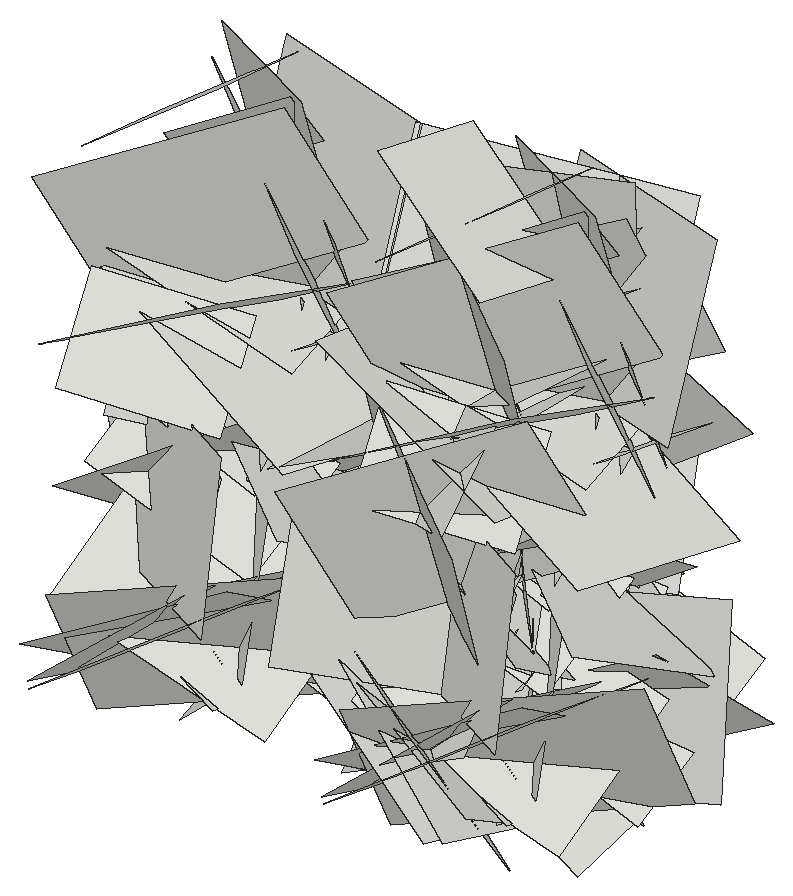
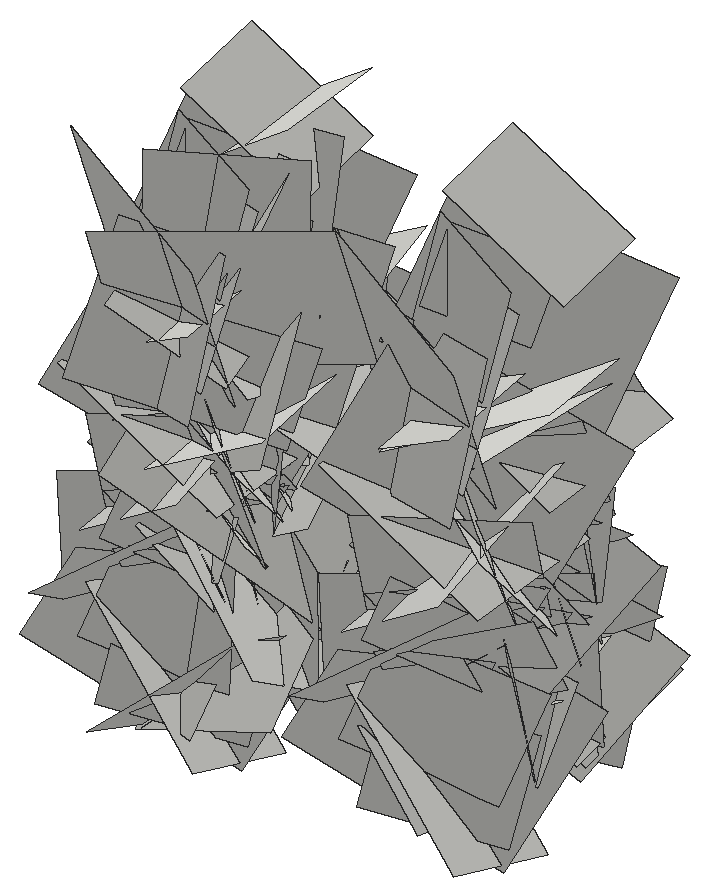
# SketchUp Ruby script. Lengths in inches.
U = 1.inch
M = Sketchup.active_model
def pt(a) = Geom::Point3d.new(a.map { |v| v * U })
def face(e, loops, mat)
  f = e.add_face(loops[0].map { |a| pt(a) })
  loops[1..].each { |l| e.add_face(l.map { |a| pt(a) }).erase! }
  f.material = f.back_material = mat if mat
  f
end
# faces: each face lists its corners as indices into pts; further lists are holes
def faces(e, pts, list, mat = nil) = list.each { |f| face(e, (f[0].is_a?(Array) ? f : [f]).map { |l| l.map { |i| pts[i] } }, mat) }
# xy, xz, yz: faces in a plane at the given z, y or x. An outline is a flat list of corners, or four numbers for a rectangle; further outlines are holes
def ring(l) = l.size == 4 ? [[l[0], l[1]], [l[2], l[1]], [l[2], l[3]], [l[0], l[3]]] : l.each_slice(2).to_a
def flat(e, list, mat, &to3) = list.each { |f| face(e, (f[0].is_a?(Array) ? f : [f]).map { |l| ring(l).map { |u, v| to3.(u, v) } }, mat) }
def xy(e, z, list, mat = nil) = flat(e, list, mat) { |x, y| [x, y, z] }
def xz(e, y, list, mat = nil) = flat(e, list, mat) { |x, z| [x, y, z] }
def yz(e, x, list, mat = nil) = flat(e, list, mat) { |y, z| [x, y, z] }
def lines(e, pts, list) = list.each { |a, b| e.add_line(pt(pts[a]), pt(pts[b])) }
# prism: a flat outline (further loops are holes) pulled along v
def prism(e, loops, v, mat = nil)
  f = face(e, loops, mat); d = Geom::Vector3d.new(v.map { |x| x * U })
  f.pushpull(f.normal.samedirection?(d) ? d.length : -d.length)
end
def box(e, o, s, mat = nil) = prism(e, [[o, [o[0] + s[0], o[1], o[2]], [o[0] + s[0], o[1] + s[1], o[2]], [o[0], o[1] + s[1], o[2]]]], [0, 0, s[2]], mat)
def at(x, y, z, deg = 0) = Geom::Transformation.translation(pt([x, y, z])) * Geom::Transformation.rotation(ORIGIN, Z_AXIS, deg.degrees)
def axes(o, x, y, z) = Geom::Transformation.new([*x, 0, *y, 0, *z, 0, *pt(o).to_a, 1])
def part(name) = M.definitions.add(name)
# library, detail: a bought-in or finely detailed component or shape, given as its bounding box
def library(name, o, s) = part(name).tap { |d| box(d.entities, o, s) }
def detail(e, o, s) = box(e.add_group.entities, o, s)
def put(e, d, t, mat = nil) = e.add_instance(d, t).tap { |i| i.material = mat if mat }
def group(e, t, mat = nil) = e.add_group.tap { |g| g.transformation = t; g.material = mat if mat }.entities
root = M.entities
c1 = part("Component\#6")
p = [[0.01,0,0],[0,3.24,4.54],[4.32,3.24,4.54],[4.33,0,0]]
faces(c1.entities,p,[[0,1,2,3]])
put(root,c1,axes([424.49,131.21,27.63],[0.2234,-0.54463,1.08834],[0.02633,1.10624,0.54877],[-1.28976,-0.07175,0.19972]))
put(root,c1,axes([420.52,131.21,27.63],[-0.2234,-0.54463,1.08834],[-0.02633,1.10624,0.54877],[1.28976,-0.07175,0.19972]))
put(root,c1,axes([410.71,134.27,30.6],[0.0256,-0.22889,-1.14247],[0.00761,-1.14266,0.22909],[1.23506,0.01178,0.02227]))
put(root,c1,axes([420.52,134.27,30.6],[0.0256,-0.22889,-1.14247],[0.00761,-1.14266,0.22909],[1.23506,0.01178,0.02227]))
put(root,c1,axes([424.49,134.27,30.6],[-0.0256,-0.22889,-1.14247],[-0.00761,-1.14266,0.22909],[-1.23506,0.01178,0.02227]))
put(root,c1,axes([420.52,134.18,33.55],[-0.07538,-0.44425,-0.62436],[0.04133,-0.62833,0.44263],[0.8112,-0.00926,-0.08057]))
put(root,c1,axes([414.68,134.18,33.55],[0.07538,-0.44425,-0.62436],[-0.04133,-0.62833,0.44263],[-0.8112,-0.00926,-0.08057]))
put(root,c1,axes([424.49,134.18,33.55],[0.07538,-0.44425,-0.62436],[-0.04133,-0.62833,0.44263],[-0.8112,-0.00926,-0.08057]))
put(root,c1,axes([410.71,134.17,21.91],[-0.00769,-1.04417,0.30366],[-0.13881,0.30229,1.03635],[1.14428,0.02965,0.12776]))
put(root,c1,axes([420.52,134.17,21.91],[-0.00769,-1.04417,0.30366],[-0.13881,0.30229,1.03635],[1.14428,0.02965,0.12776]))
put(root,c1,axes([424.49,134.17,21.91],[0.00769,-1.04417,0.30366],[0.13881,0.30229,1.03635],[-1.14428,0.02965,0.12776]))
put(root,c1,axes([410.71,134.58,22.11],[0.07114,-1.22092,0.271],[-0.02912,0.26988,1.2227],[1.32535,0.07146,0.01232]))
put(root,c1,axes([424.49,134.58,22.11],[-0.07114,-1.22092,0.271],[0.02912,0.26988,1.2227],[-1.32535,0.07146,0.01232]))
put(root,c1,axes([420.52,134.58,22.11],[0.07114,-1.22092,0.271],[-0.02912,0.26988,1.2227],[1.32535,0.07146,0.01232]))
put(root,c1,axes([410.71,134.42,21.5625],[-0.1234,-1.02964,0.56694],[0.11588,0.55776,1.03542],[1.24053,-0.15452,-0.04032]))
put(root,c1,axes([420.52,134.42,21.5625],[-0.1234,-1.02964,0.56694],[0.11588,0.55776,1.03542],[1.24053,-0.15452,-0.04032]))
put(root,c1,axes([424.49,134.42,21.5625],[0.1234,-1.02964,0.56694],[-0.11588,0.55776,1.03542],[-1.24053,-0.15452,-0.04032]))
put(root,c1,axes([410.71,132.49,21.15],[0.19066,-0.73145,1.17679],[0.11238,1.19045,0.72374],[1.46442,0.00387,-0.20876]))
put(root,c1,axes([420.52,132.49,21.15],[0.19066,-0.73145,1.17679],[0.11238,1.19045,0.72374],[1.46442,0.00387,-0.20876]))
put(root,c1,axes([424.49,132.49,21.15],[-0.19066,-0.73145,1.17679],[-0.11238,1.19045,0.72374],[-1.46442,0.00387,-0.20876]))
put(root,c1,axes([420.52,134.6875,22.2],[-0.10426,-0.66856,0.17597],[0.06243,0.169,0.67497],[0.73015,-0.10992,-0.03258]))
put(root,c1,axes([414.68,134.6875,22.2],[0.10426,-0.66856,0.17597],[-0.06243,0.169,0.67497],[-0.73015,-0.10992,-0.03258]))
put(root,c1,axes([424.49,134.6875,22.2],[0.10426,-0.66856,0.17597],[-0.06243,0.169,0.67497],[-0.73015,-0.10992,-0.03258]))
put(root,c1,axes([414.68,131.06,25.92],[0.11704,0.23417,0.88186],[0.10525,0.87993,-0.24609],[-0.96142,0.12483,0.08041]))
put(root,c1,axes([420.52,131.06,25.92],[-0.11704,0.23417,0.88186],[-0.10525,0.87993,-0.24609],[0.96142,0.12483,0.08041]))
put(root,c1,axes([424.49,131.06,25.92],[0.11704,0.23417,0.88186],[0.10525,0.87993,-0.24609],[-0.96142,0.12483,0.08041]))
put(root,c1,axes([410.71,130.54,25.39],[0.14552,0.87979,0.74939],[0.0105,0.75374,-0.8867],[1.22498,-0.11098,-0.08143]))
put(root,c1,axes([420.52,130.54,25.39],[0.14552,0.87979,0.74939],[0.0105,0.75374,-0.8867],[1.22498,-0.11098,-0.08143]))
put(root,c1,axes([424.49,130.54,25.39],[-0.14552,0.87979,0.74939],[-0.0105,0.75374,-0.8867],[-1.22498,-0.11098,-0.08143]))
put(root,c1,axes([410.71,135.84,31.22],[-0.16391,-1.12855,0.28901],[0.13375,0.27361,1.13591],[1.2276,-0.1805,-0.08517]))
put(root,c1,axes([420.52,135.84,31.22],[-0.16391,-1.12855,0.28901],[0.13375,0.27361,1.13591],[1.2276,-0.1805,-0.08517]))
put(root,c1,axes([424.49,135.84,31.22],[0.16391,-1.12855,0.28901],[-0.13375,0.27361,1.13591],[-1.2276,-0.1805,-0.08517]))
put(root,c1,axes([410.71,135.18,37.85],[0.05885,-0.83818,0.13983],[-0.03078,0.13818,0.83979],[0.90022,0.05952,0.01957]))
put(root,c1,axes([420.52,135.18,37.85],[0.05885,-0.83818,0.13983],[-0.03078,0.13818,0.83979],[0.90022,0.05952,0.01957]))
put(root,c1,axes([424.49,135.18,37.85],[-0.05885,-0.83818,0.13983],[0.03078,0.13818,0.83979],[-0.90022,0.05952,0.01957]))
put(root,c1,axes([410.71,133.37,32.625],[-0.2234,-0.54463,1.08834],[-0.02633,1.10624,0.54877],[1.28976,-0.07175,0.19972]))
put(root,c1,axes([424.49,133.37,32.625],[0.2234,-0.54463,1.08834],[0.02633,1.10624,0.54877],[-1.28976,-0.07175,0.19972]))
put(root,c1,axes([420.52,133.37,32.625],[-0.2234,-0.54463,1.08834],[-0.02633,1.10624,0.54877],[1.28976,-0.07175,0.19972]))
put(root,c1,axes([410.71,131.97,28.78],[0.10091,0.74431,0.53228],[-0.01265,0.53611,-0.74754],[0.96987,-0.07045,-0.06513]))
put(root,c1,axes([420.52,131.97,28.78],[0.10091,0.74431,0.53228],[-0.01265,0.53611,-0.74754],[0.96987,-0.07045,-0.06513]))
put(root,c1,axes([424.49,131.97,28.78],[-0.10091,0.74431,0.53228],[0.01265,0.53611,-0.74754],[-0.96987,-0.07045,-0.06513]))
put(root,c1,axes([414.68,136.41,29.65],[0.07813,-0.63244,-0.26103],[0.10098,-0.25049,0.63382],[-0.71818,-0.10402,0.06072]))
put(root,c1,axes([420.52,136.41,29.65],[-0.07813,-0.63244,-0.26103],[-0.10098,-0.25049,0.63382],[0.71818,-0.10402,0.06072]))
put(root,c1,axes([424.49,136.41,29.65],[0.07813,-0.63244,-0.26103],[0.10098,-0.25049,0.63382],[-0.71818,-0.10402,0.06072]))
put(root,c1,axes([410.71,134.54,24.9375],[0.02484,0.40022,-0.64969],[0.07983,-0.64803,-0.39648],[0.8049,0.05192,0.05937]))
put(root,c1,axes([420.52,134.54,24.9375],[0.02484,0.40022,-0.64969],[0.07983,-0.64803,-0.39648],[0.8049,0.05192,0.05937]))
put(root,c1,axes([424.49,134.54,24.9375],[-0.02484,0.40022,-0.64969],[-0.07983,-0.64803,-0.39648],[-0.8049,0.05192,0.05937]))
put(root,c1,axes([410.71,136.25,25.03],[-0.1909,-1.05424,0.65515],[0.04228,0.65676,1.06778],[1.31502,-0.17416,0.06077]))
put(root,c1,axes([420.52,136.25,25.03],[-0.1909,-1.05424,0.65515],[0.04228,0.65676,1.06778],[1.31502,-0.17416,0.06077]))
put(root,c1,axes([424.49,136.25,25.03],[0.1909,-1.05424,0.65515],[-0.04228,0.65676,1.06778],[-1.31502,-0.17416,0.06077]))
put(root,c1,axes([410.71,132.63,34.3],[0.186,1.33026,-0.17859],[0.24164,-0.20703,-1.31812],[1.40205,-0.1408,0.25087]))
put(root,c1,axes([420.52,132.63,34.3],[0.186,1.33026,-0.17859],[0.24164,-0.20703,-1.31812],[1.40205,-0.1408,0.25087]))
put(root,c1,axes([424.49,132.63,34.3],[-0.186,1.33026,-0.17859],[-0.24164,-0.20703,-1.31812],[-1.40205,-0.1408,0.25087]))
put(root,c1,axes([410.71,132.79,29.8],[0.04873,0.29435,0.84438],[-0.1159,0.841,-0.28722],[0.94075,0.08836,-0.07912]))
put(root,c1,axes([424.49,132.79,29.8],[-0.04873,0.29435,0.84438],[0.1159,0.841,-0.28722],[-0.94075,0.08836,-0.07912]))
put(root,c1,axes([420.52,132.79,29.8],[0.04873,0.29435,0.84438],[-0.1159,0.841,-0.28722],[0.94075,0.08836,-0.07912]))
put(root,c1,axes([410.71,137.68,26.93],[0.04018,-0.30696,-1.06119],[-0.15368,-1.05402,0.2997],[1.16085,-0.12891,0.07641]))
put(root,c1,axes([420.52,137.68,26.93],[0.04018,-0.30696,-1.06119],[-0.15368,-1.05402,0.2997],[1.16085,-0.12891,0.07641]))
put(root,c1,axes([424.49,137.68,26.93],[-0.04018,-0.30696,-1.06119],[0.15368,-1.05402,0.2997],[-1.16085,-0.12891,0.07641]))
put(root,c1,axes([410.71,133.57,26.39],[-0.0097,-0.16576,1.00827],[-0.11893,1.00238,0.16377],[1.07657,0.10924,0.02717]))
put(root,c1,axes([420.52,133.57,26.39],[-0.0097,-0.16576,1.00827],[-0.11893,1.00238,0.16377],[1.07657,0.10924,0.02717]))
put(root,c1,axes([424.49,133.57,26.39],[0.0097,-0.16576,1.00827],[0.11893,1.00238,0.16377],[-1.07657,0.10924,0.02717]))
put(root,c1,axes([420.52,135.55,39.48],[0.03347,0.37514,-0.47819],[-0.05412,-0.47551,-0.37641],[0.64197,-0.05964,-0.0068]))
put(root,c1,axes([414.68,135.55,39.48],[-0.03347,0.37514,-0.47819],[0.05412,-0.47551,-0.37641],[-0.64197,-0.05964,-0.0068]))
put(root,c1,axes([424.49,135.55,39.48],[-0.03347,0.37514,-0.47819],[0.05412,-0.47551,-0.37641],[-0.64197,-0.05964,-0.0068]))
put(root,c1,axes([410.71,132.63,35],[-0.22269,1.01925,0.0867],[0.15354,0.11726,-1.02752],[1.07338,0.19468,0.16497]))
put(root,c1,axes([420.52,132.63,35],[-0.22269,1.01925,0.0867],[0.15354,0.11726,-1.02752],[1.07338,0.19468,0.16497]))
put(root,c1,axes([424.49,132.63,35],[0.22269,1.01925,0.0867],[-0.15354,0.11726,-1.02752],[-1.07338,0.19468,0.16497]))
put(root,c1,axes([410.71,133.32,22.11],[0.03082,0.0656,1.39488],[-0.001,1.39518,-0.0656],[1.48021,-0.00042,-0.02909]))
put(root,c1,axes([420.52,133.32,22.11],[0.03082,0.0656,1.39488],[-0.001,1.39518,-0.0656],[1.48021,-0.00042,-0.02909]))
put(root,c1,axes([424.49,133.32,22.11],[-0.03082,0.0656,1.39488],[0.001,1.39518,-0.0656],[-1.48021,-0.00042,-0.02909]))
put(root,c1,axes([410.71,133.77,26.39],[-0.09062,0.64279,0.71838],[0.13606,0.72237,-0.63108],[1.01272,-0.03954,0.14907]))
put(root,c1,axes([420.52,133.77,26.39],[-0.09062,0.64279,0.71838],[0.13606,0.72237,-0.63108],[1.01272,-0.03954,0.14907]))
put(root,c1,axes([424.49,133.77,26.39],[0.09062,0.64279,0.71838],[-0.13606,0.72237,-0.63108],[-1.01272,-0.03954,0.14907]))
put(root,c1,axes([410.71,139.12,30.95],[-0.15428,-0.64193,-0.79007],[0.04846,-0.80142,0.64273],[1.07797,-0.05585,-0.14197]))
put(root,c1,axes([420.52,139.12,30.95],[-0.15428,-0.64193,-0.79007],[0.04846,-0.80142,0.64273],[1.07797,-0.05585,-0.14197]))
put(root,c1,axes([424.49,139.12,30.95],[0.15428,-0.64193,-0.79007],[-0.04846,-0.80142,0.64273],[-1.07797,-0.05585,-0.14197]))
put(root,c1,axes([410.71,134.64,27.51],[0.11331,0.92563,-0.03565],[-0.09128,-0.0258,-0.92812],[0.97764,-0.10969,-0.08252]))
put(root,c1,axes([420.52,134.64,27.51],[0.11331,0.92563,-0.03565],[-0.09128,-0.0258,-0.92812],[0.97764,-0.10969,-0.08252]))
put(root,c1,axes([424.49,134.64,27.51],[-0.11331,0.92563,-0.03565],[0.09128,-0.0258,-0.92812],[-0.97764,-0.10969,-0.08252]))
put(root,c1,axes([410.71,135.17,32.61],[0.12448,1.21649,-0.63228],[-0.14654,-0.62086,-1.22019],[1.44585,-0.16766,-0.06923]))
put(root,c1,axes([420.52,135.17,32.61],[0.12448,1.21649,-0.63228],[-0.14654,-0.62086,-1.22019],[1.44585,-0.16766,-0.06923]))
put(root,c1,axes([424.49,135.17,32.61],[-0.12448,1.21649,-0.63228],[0.14654,-0.62086,-1.22019],[-1.44585,-0.16766,-0.06923]))
put(root,c1,axes([410.71,136.8125,27.97],[-0.23976,-0.84366,1.03424],[-0.08712,1.0558,0.84327],[1.41209,-0.07811,0.22763]))
put(root,c1,axes([420.52,136.8125,27.97],[-0.23976,-0.84366,1.03424],[-0.08712,1.0558,0.84327],[1.41209,-0.07811,0.22763]))
put(root,c1,axes([424.49,136.8125,27.97],[0.23976,-0.84366,1.03424],[0.08712,1.0558,0.84327],[-1.41209,-0.07811,0.22763]))
put(root,c1,axes([410.71,132.97,26.35],[0.04012,1.17129,0.65858],[-0.12839,0.65914,-1.16531],[1.41857,0.02653,-0.1241]))
put(root,c1,axes([420.52,132.97,26.35],[0.04012,1.17129,0.65858],[-0.12839,0.65914,-1.16531],[1.41857,0.02653,-0.1241]))
put(root,c1,axes([424.49,132.97,26.35],[-0.04012,1.17129,0.65858],[0.12839,0.65914,-1.16531],[-1.41857,0.02653,-0.1241]))
put(root,c1,axes([410.71,137.29,38.52],[-0.00887,0.62519,-1.13199],[-0.07674,-1.13046,-0.62381],[1.3686,-0.05933,-0.04231]))
put(root,c1,axes([420.52,137.29,38.52],[-0.00887,0.62519,-1.13199],[-0.07674,-1.13046,-0.62381],[1.3686,-0.05933,-0.04231]))
put(root,c1,axes([424.49,137.29,38.52],[0.00887,0.62519,-1.13199],[0.07674,-1.13046,-0.62381],[-1.3686,-0.05933,-0.04231]))
put(root,c1,axes([414.68,134.33,29.51],[0.0444,0.3698,0.86525],[0.11423,0.85852,-0.37214],[-0.99086,0.11554,-0.00413]))
put(root,c1,axes([420.52,134.33,29.51],[-0.0444,0.3698,0.86525],[-0.11423,0.85852,-0.37214],[0.99086,0.11554,-0.00413]))
put(root,c1,axes([424.49,134.33,29.51],[0.0444,0.3698,0.86525],[0.11423,0.85852,-0.37214],[-0.99086,0.11554,-0.00413]))
put(root,c1,axes([410.71,139.23,29.07],[-0.06497,-1.13195,0.1646],[0.10003,0.15928,1.13044],[1.20835,-0.07404,-0.08473]))
put(root,c1,axes([420.52,139.23,29.07],[-0.06497,-1.13195,0.1646],[0.10003,0.15928,1.13044],[1.20835,-0.07404,-0.08473]))
put(root,c1,axes([424.49,139.23,29.07],[0.06497,-1.13195,0.1646],[-0.10003,0.15928,1.13044],[-1.20835,-0.07404,-0.08473]))
put(root,c1,axes([410.71,137.68,39.44],[0.12024,0.16456,-0.83242],[0.12638,-0.83458,-0.14874],[0.89051,0.09622,0.13351]))
put(root,c1,axes([420.52,137.68,39.44],[0.12024,0.16456,-0.83242],[0.12638,-0.83458,-0.14874],[0.89051,0.09622,0.13351]))
put(root,c1,axes([424.49,137.68,39.44],[-0.12024,0.16456,-0.83242],[-0.12638,-0.83458,-0.14874],[-0.89051,0.09622,0.13351]))
put(root,c1,axes([410.71,138.04,20.07],[-0.12016,-0.9858,0.86253],[0.12902,0.85408,0.99214],[1.38246,-0.16539,-0.01763]))
put(root,c1,axes([424.49,138.04,20.07],[0.12016,-0.9858,0.86253],[-0.12902,0.85408,0.99214],[-1.38246,-0.16539,-0.01763]))
put(root,c1,axes([420.52,138.04,20.07],[-0.12016,-0.9858,0.86253],[0.12902,0.85408,0.99214],[1.38246,-0.16539,-0.01763]))
put(root,c1,axes([420.52,139.13,26.61],[-0.02912,-0.4172,-0.72752],[-0.02466,-0.72725,0.41792],[0.88863,-0.03385,-0.01224]))
put(root,c1,axes([414.68,139.13,26.61],[0.02912,-0.4172,-0.72752],[0.02466,-0.72725,0.41792],[-0.88863,-0.03385,-0.01224]))
put(root,c1,axes([424.49,139.13,26.61],[0.02912,-0.4172,-0.72752],[0.02466,-0.72725,0.41792],[-0.88863,-0.03385,-0.01224]))
put(root,c1,axes([410.71,140.34,20.98],[0.05969,-1.08852,-0.33352],[-0.17093,-0.33819,1.07653],[1.19461,0.00599,0.1707]))
put(root,c1,axes([424.49,140.34,20.98],[-0.05969,-1.08852,-0.33352],[0.17093,-0.33819,1.07653],[-1.19461,0.00599,0.1707]))
put(root,c1,axes([420.52,140.34,20.98],[0.05969,-1.08852,-0.33352],[-0.17093,-0.33819,1.07653],[1.19461,0.00599,0.1707]))
put(root,c1,axes([420.52,137.74,29.49],[-0.05063,0.39266,-0.56355],[-0.15447,-0.55784,-0.37633],[0.71149,-0.09317,-0.12181]))
put(root,c1,axes([414.68,137.74,29.49],[0.05063,0.39266,-0.56355],[0.15447,-0.55784,-0.37633],[-0.71149,-0.09317,-0.12181]))
put(root,c1,axes([424.49,137.74,29.49],[0.05063,0.39266,-0.56355],[0.15447,-0.55784,-0.37633],[-0.71149,-0.09317,-0.12181]))
put(root,c1,axes([410.71,135.78,27.7],[-0.08438,0.31612,0.89331],[0.15155,0.8902,-0.30228],[0.99295,-0.109,0.12205]))
put(root,c1,axes([420.52,135.78,27.7],[-0.08438,0.31612,0.89331],[0.15155,0.8902,-0.30228],[0.99295,-0.109,0.12205]))
put(root,c1,axes([424.49,135.78,27.7],[0.08438,0.31612,0.89331],[-0.15155,0.8902,-0.30228],[-0.99295,-0.109,0.12205]))
put(root,c1,axes([410.71,140.4,37.84],[-0.00777,-0.46206,-1.23937],[0.21731,-1.22481,0.45542],[1.38512,0.18957,-0.0784]))
put(root,c1,axes([424.49,140.4,37.84],[0.00777,-0.46206,-1.23937],[-0.21731,-1.22481,0.45542],[-1.38512,0.18957,-0.0784]))
put(root,c1,axes([420.52,140.4,37.84],[-0.00777,-0.46206,-1.23937],[0.21731,-1.22481,0.45542],[1.38512,0.18957,-0.0784]))
put(root,c1,axes([420.52,138.35,27.1],[-0.19626,0.31166,-0.79897],[0.02742,-0.81497,-0.3239],[0.90864,0.09191,-0.1628]))
put(root,c1,axes([414.68,138.35,27.1],[0.19626,0.31166,-0.79897],[-0.02742,-0.81497,-0.3239],[-0.90864,0.09191,-0.1628]))
put(root,c1,axes([424.49,138.35,27.1],[0.19626,0.31166,-0.79897],[-0.02742,-0.81497,-0.3239],[-0.90864,0.09191,-0.1628]))
put(root,c1,axes([410.71,137.01,36.4],[0.10049,0.69541,-0.2411],[0.01368,-0.24463,-0.7005],[0.78006,-0.08529,0.04335]))
put(root,c1,axes([420.52,137.01,36.4],[0.10049,0.69541,-0.2411],[0.01368,-0.24463,-0.7005],[0.78006,-0.08529,0.04335]))
put(root,c1,axes([424.49,137.01,36.4],[-0.10049,0.69541,-0.2411],[-0.01368,-0.24463,-0.7005],[-0.78006,-0.08529,0.04335]))
put(root,c1,axes([410.71,137.76,20.74],[0.07875,-0.43706,0.66864],[-0.02301,0.67018,0.44047],[0.84643,0.05888,-0.05024]))
put(root,c1,axes([420.52,137.76,20.74],[0.07875,-0.43706,0.66864],[-0.02301,0.67018,0.44047],[0.84643,0.05888,-0.05024]))
put(root,c1,axes([424.49,137.76,20.74],[-0.07875,-0.43706,0.66864],[0.02301,0.67018,0.44047],[-0.84643,0.05888,-0.05024]))
put(root,c1,axes([410.71,138.81,37.71],[-0.08326,0.50336,-1.07522],[-0.02589,-1.07803,-0.50289],[1.25818,0.01113,-0.0815]))
put(root,c1,axes([420.52,138.81,37.71],[-0.08326,0.50336,-1.07522],[-0.02589,-1.07803,-0.50289],[1.25818,0.01113,-0.0815]))
put(root,c1,axes([424.49,138.81,37.71],[0.08326,0.50336,-1.07522],[0.02589,-1.07803,-0.50289],[-1.25818,0.01113,-0.0815]))
put(root,c1,axes([420.52,136.62,23.89],[-0.08859,0.63974,0.04756],[-0.12242,0.03217,-0.63572],[0.66888,0.09062,-0.11005]))
put(root,c1,axes([414.68,136.62,23.89],[0.08859,0.63974,0.04756],[0.12242,0.03217,-0.63572],[-0.66888,0.09062,-0.11005]))
